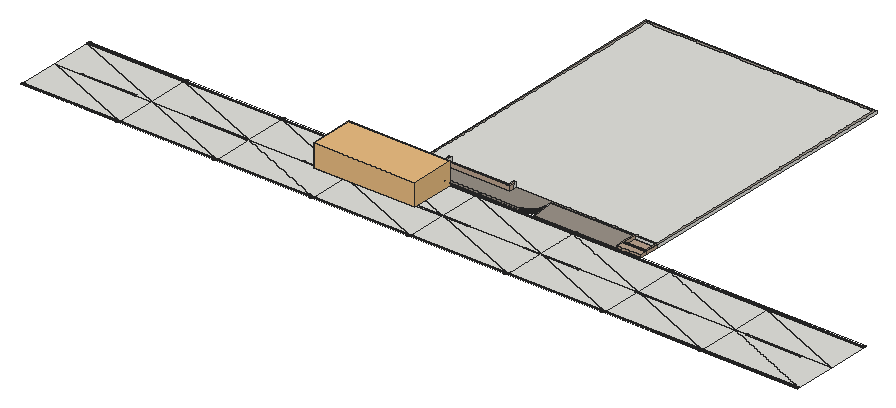
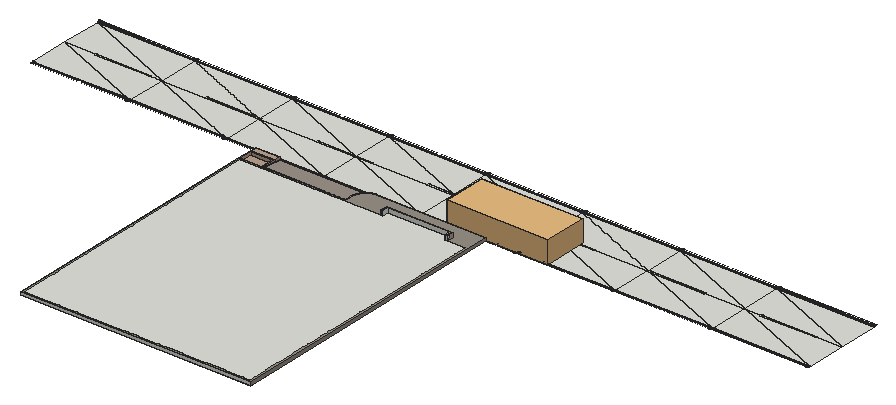
# SketchUp Ruby script. Lengths in inches.
U = 1.inch
M = Sketchup.active_model
def pt(a) = Geom::Point3d.new(a.map { |v| v * U })
def face(e, loops, mat)
  f = e.add_face(loops[0].map { |a| pt(a) })
  loops[1..].each { |l| e.add_face(l.map { |a| pt(a) }).erase! }
  f.material = f.back_material = mat if mat
  f
end
# faces: each face lists its corners as indices into pts; further lists are holes
def faces(e, pts, list, mat = nil) = list.each { |f| face(e, (f[0].is_a?(Array) ? f : [f]).map { |l| l.map { |i| pts[i] } }, mat) }
# xy, xz, yz: faces in a plane at the given z, y or x. An outline is a flat list of corners, or four numbers for a rectangle; further outlines are holes
def ring(l) = l.size == 4 ? [[l[0], l[1]], [l[2], l[1]], [l[2], l[3]], [l[0], l[3]]] : l.each_slice(2).to_a
def flat(e, list, mat, &to3) = list.each { |f| face(e, (f[0].is_a?(Array) ? f : [f]).map { |l| ring(l).map { |u, v| to3.(u, v) } }, mat) }
def xy(e, z, list, mat = nil) = flat(e, list, mat) { |x, y| [x, y, z] }
def xz(e, y, list, mat = nil) = flat(e, list, mat) { |x, z| [x, y, z] }
def yz(e, x, list, mat = nil) = flat(e, list, mat) { |y, z| [x, y, z] }
def lines(e, pts, list) = list.each { |a, b| e.add_line(pt(pts[a]), pt(pts[b])) }
# prism: a flat outline (further loops are holes) pulled along v
def prism(e, loops, v, mat = nil)
  f = face(e, loops, mat); d = Geom::Vector3d.new(v.map { |x| x * U })
  f.pushpull(f.normal.samedirection?(d) ? d.length : -d.length)
end
def box(e, o, s, mat = nil) = prism(e, [[o, [o[0] + s[0], o[1], o[2]], [o[0] + s[0], o[1] + s[1], o[2]], [o[0], o[1] + s[1], o[2]]]], [0, 0, s[2]], mat)
def at(x, y, z, deg = 0) = Geom::Transformation.translation(pt([x, y, z])) * Geom::Transformation.rotation(ORIGIN, Z_AXIS, deg.degrees)
def axes(o, x, y, z) = Geom::Transformation.new([*x, 0, *y, 0, *z, 0, *pt(o).to_a, 1])
def part(name) = M.definitions.add(name)
# library, detail: a bought-in or finely detailed component or shape, given as its bounding box
def library(name, o, s) = part(name).tap { |d| box(d.entities, o, s) }
def detail(e, o, s) = box(e.add_group.entities, o, s)
def put(e, d, t, mat = nil) = e.add_instance(d, t).tap { |i| i.material = mat if mat }
def group(e, t, mat = nil) = e.add_group.tap { |g| g.transformation = t; g.material = mat if mat }.entities
root = M.entities
M.materials.add("Sand Stones 01 100cm").color = [188, 164, 143]
M.materials.add("Tiles L02 200cm").color = [152, 144, 134]
c1 = library("Car 033",[-43.24,-98.19,-1.29],[86.48,201.64,57.79])
xy(root,0.19,[[0,119.84,0.61,119.84,0,120.23],[0.61,119.84,0.61,120.23,0,120.23],[0,281.6,0.66,281.6,0,281.84],[0.66,281.6,0.66,281.84,0,281.84],[0,281.84,0.66,281.84,0,285.35],
  [0.66,281.84,0.66,285.35,0,285.35],[0,285.35,0.66,285.35,0,285.61],[0.66,285.35,0.66,285.61,0,285.61]])
xz(root,115.97,[[0,-0.1,0,0.09,192.375,0.11],[0,-0.1,192.375,0.11,192.375,-0.07],[192.375,-0.07,192.375,0.11,384.75,-0.05],[384.75,-0.05,192.375,0.11,384.75,0.13],[384.75,-0.05,384.75,0.13,577.125,-0.03],
  [577.125,-0.03,384.75,0.13,577.125,0.15],[577.125,-0.03,577.125,0.15,769.5,-0.01],[769.5,-0.01,577.125,0.15,769.5,0.18],[769.5,-0.01,769.5,0.18,961.88,0.02],[961.88,0.02,769.5,0.18,961.88,0.2],
  [961.88,0.02,961.88,0.2,1154.25,0.04],[1154.25,0.04,961.88,0.2,1154.25,0.22],[1154.25,0.04,1154.25,0.22,1346.63,0.0625],[1346.63,0.0625,1154.25,0.22,1346.63,0.24],[1346.63,0.0625,1346.63,0.24,1539,0.27],
  [1346.63,0.0625,1539,0.27,1539,0.08]])
xz(root,116.08,[[0,-0.1,0.61,-0.1,0,0.09],[0.61,-0.1,0.61,0.09,0,0.09],[0.61,-0.1,192.375,-0.07,0.61,0.09],[192.375,-0.07,192.375,0.11,0.61,0.09],[192.375,-0.07,384.75,-0.05,384.75,0.13],
  [192.375,-0.07,384.75,0.13,192.375,0.11],[384.75,-0.05,577.125,-0.03,577.125,0.15],[384.75,-0.05,577.125,0.15,384.75,0.13],[577.125,-0.03,769.5,-0.01,769.5,0.18],[577.125,-0.03,769.5,0.18,577.125,0.15],
  [769.5,-0.01,961.875,0.02,961.875,0.2],[769.5,-0.01,961.875,0.2,769.5,0.18],[961.875,0.02,1154.25,0.04,1154.25,0.22],[961.875,0.02,1154.25,0.22,961.875,0.2],[1154.25,0.04,1346.625,0.0625,1346.625,0.24],
  [1154.25,0.04,1346.625,0.24,1154.25,0.22],[1346.625,0.0625,1538.36,0.08,1346.625,0.24],[1538.36,0.08,1538.36,0.27,1346.625,0.24],[1538.36,0.08,1539,0.08,1538.36,0.27],[1539,0.08,1539,0.27,1538.36,0.27]])
xz(root,120.55,[[0,-1.53,0,-0.19,0.61,-0.19],[0,-1.53,0.61,-0.19,0.61,-1.53],[0.61,-1.53,0.61,-0.19,192.375,-0.17],[0.61,-1.53,192.375,-0.17,192.375,-1.51],[192.375,-1.51,192.375,-0.17,384.75,-0.15],
  [192.375,-1.51,384.75,-0.15,384.75,-1.49],[384.75,-1.49,384.75,-0.15,577.125,-0.13],[384.75,-1.49,577.125,-0.13,577.125,-1.46],[577.125,-1.46,577.125,-0.13,769.5,-1.44],[769.5,-1.44,577.125,-0.13,769.5,-0.1],
  [769.5,-1.44,769.5,-0.1,961.875,-0.08],[769.5,-1.44,961.875,-0.08,961.875,-1.42],[961.875,-1.42,1154.25,-0.06,1154.25,-1.4],[961.875,-1.42,961.875,-0.08,1154.25,-0.06],[1154.25,-1.4,1154.25,-0.06,1346.625,-0.04],
  [1154.25,-1.4,1346.625,-0.04,1346.63,-1.375],[1346.63,-1.375,1346.625,-0.04,1538.36,-0.01],[1346.63,-1.375,1538.36,-0.01,1538.36,-1.35],[1538.36,-1.35,1538.36,-0.01,1539,-0.01],[1538.36,-1.35,1539,-0.01,1539,-1.35],
  [0,-0.19,0,-0.01,0.61,-0.01],[0,-0.19,0.61,-0.01,0.61,-0.19],[0.61,-0.19,0.61,-0.01,192.375,0.01],[0.61,-0.19,192.375,0.01,192.375,-0.17],[192.375,-0.17,192.375,0.01,384.75,-0.15],
  [384.75,-0.15,192.375,0.01,384.75,0.03],[384.75,-0.15,384.75,0.03,577.125,-0.13],[577.125,-0.13,384.75,0.03,577.125,0.06],[577.125,-0.13,577.125,0.06,769.5,0.08],[577.125,-0.13,769.5,0.08,769.5,-0.1],
  [769.5,-0.1,769.5,0.08,961.875,-0.08],[961.875,-0.08,769.5,0.08,961.875,0.1],[961.875,-0.08,961.875,0.1,1154.25,-0.06],[1154.25,-0.06,961.875,0.1,1154.25,0.125],[1154.25,-0.06,1154.25,0.125,1346.625,-0.04],
  [1346.625,-0.04,1154.25,0.125,1346.625,0.15],[1346.625,-0.04,1346.625,0.15,1538.36,0.17],[1346.625,-0.04,1538.36,0.17,1538.36,-0.01],[1538.36,-0.01,1538.36,0.17,1539,0.17],[1538.36,-0.01,1539,0.17,1539,-0.01]])
xz(root,281.28,[[0,-1.53,0.66,-1.53,0,-0.31],[0.66,-1.53,0.66,-0.31,0,-0.31],[0.66,-1.53,192.375,-1.51,0.66,-0.31],[192.375,-1.51,192.375,-0.28,0.66,-0.31],[192.375,-1.51,384.75,-0.26,192.375,-0.28],
  [192.375,-1.51,384.75,-1.49,384.75,-0.26],[384.75,-1.49,577.125,-0.24,384.75,-0.26],[384.75,-1.49,577.125,-1.47,577.125,-0.24],[577.125,-1.47,769.5,-1.44,577.125,-0.24],[769.5,-1.44,769.5,-0.22,577.125,-0.24],
  [769.5,-1.44,961.875,-0.19,769.5,-0.22],[769.5,-1.44,961.875,-1.42,961.875,-0.19],[961.875,-1.42,1154.25,-0.17,961.875,-0.19],[961.875,-1.42,1154.25,-1.4,1154.25,-0.17],[1154.25,-1.4,1346.63,-0.15,1154.25,-0.17],
  [1154.25,-1.4,1346.63,-1.38,1346.63,-0.15],[1346.63,-1.38,1538.23,-1.35,1346.63,-0.15],[1538.23,-1.35,1538.23,-0.125,1346.63,-0.15],[1538.23,-1.35,1539,-1.35,1538.23,-0.125],[1539,-1.35,1539,-0.125,1538.23,-0.125],
  [0,-0.31,0.66,-0.31,0,-0.01],[0.66,-0.31,0.66,-0.01,0,-0.01],[0.66,-0.31,192.375,-0.28,0.66,-0.01],[192.375,-0.28,192.375,0.01,0.66,-0.01],[192.375,-0.28,384.75,-0.26,192.375,0.01],
  [384.75,-0.26,384.75,0.03,192.375,0.01],[384.75,-0.26,577.125,-0.24,384.75,0.03],[577.125,-0.24,577.125,0.06,384.75,0.03],[577.125,-0.24,769.5,-0.22,769.5,0.08],[577.125,-0.24,769.5,0.08,577.125,0.06],
  [769.5,-0.22,961.875,-0.19,769.5,0.08],[961.875,-0.19,961.875,0.1,769.5,0.08],[961.875,-0.19,1154.25,-0.17,961.875,0.1],[1154.25,-0.17,1154.25,0.12,961.875,0.1],[1154.25,-0.17,1346.63,-0.15,1154.25,0.12],
  [1346.63,-0.15,1346.63,0.15,1154.25,0.12],[1346.63,-0.15,1538.23,-0.125,1346.63,0.15],[1538.23,-0.125,1538.23,0.17,1346.63,0.15],[1538.23,-0.125,1539,-0.125,1538.23,0.17],[1539,-0.125,1539,0.17,1538.23,0.17]])
xz(root,285.75,[[0,-0.12,0,0.08,0.66,0.08],[0,-0.12,0.66,0.08,0.66,-0.12],[0.66,-0.12,0.66,0.08,192.375,0.1],[0.66,-0.12,192.375,0.1,192.375,-0.1],[192.375,-0.1,192.375,0.1,384.75,-0.08],
  [384.75,-0.08,192.375,0.1,384.75,0.125],[384.75,-0.08,384.75,0.125,577.125,-0.05],[577.125,-0.05,384.75,0.125,577.125,0.15],[577.125,-0.05,577.125,0.15,769.5,-0.03],[769.5,-0.03,577.125,0.15,769.5,0.17],
  [769.5,-0.03,769.5,0.17,961.875,-0.01],[961.875,-0.01,769.5,0.17,961.875,0.19],[961.875,-0.01,961.875,0.19,1154.25,0.01],[1154.25,0.01,961.875,0.19,1154.25,0.22],[1154.25,0.01,1154.25,0.22,1346.63,0.04],
  [1346.63,0.04,1154.25,0.22,1346.625,0.24],[1346.63,0.04,1346.625,0.24,1538.23,0.26],[1346.63,0.04,1538.23,0.26,1538.23,0.06],[1538.23,0.06,1538.23,0.26,1539,0.26],[1538.23,0.06,1539,0.26,1539,0.06]])
p = [[0,200.91,-1.53],[0,120.55,-1.53],[192.375,120.55,-1.51],[192.375,200.91,-1.51],[384.75,120.55,-1.49],[384.75,200.91,-1.49],
  [577.125,120.55,-1.46],[577.125,200.91,-1.47],[769.5,120.55,-1.44],[769.5,200.91,-1.44],[161.27,199.56,-1.51],[161.27,202.27,-1.51],
  [51.47,202.27,-1.52],[51.47,199.56,-1.52],[380.88,199.56,-1.48],[380.88,202.27,-1.48],[271.08,202.27,-1.49],[271.08,199.56,-1.49],
  [600.49,199.56,-1.46],[600.49,202.27,-1.46],[490.6875,202.27,-1.47],[490.6875,199.56,-1.47],[0,281.28,-1.53],[192.375,281.28,-1.51],
  [384.75,281.28,-1.49],[577.125,281.28,-1.47],[769.5,281.28,-1.44],[961.875,120.55,-1.42],[961.875,200.91,-1.42],[1154.25,120.55,-1.4],
  [1154.25,200.91,-1.4],[1346.63,120.55,-1.375],[1346.63,200.91,-1.375],[1539,120.55,-1.35],[1539,200.91,-1.35],[820.1,199.56,-1.43],
  [820.1,202.27,-1.43],[710.3,202.27,-1.44],[710.3,199.56,-1.44],[1039.71,199.56,-1.4],[1039.71,202.27,-1.4],[929.91,202.27,-1.42],
  [929.91,199.56,-1.42],[1259.32,199.56,-1.38],[1259.32,202.27,-1.38],[1149.52,202.27,-1.39],[1149.52,199.56,-1.39],[1478.93,199.56,-1.35],
  [1478.93,202.27,-1.35],[1369.13,202.27,-1.37],[1369.13,199.56,-1.37],[961.875,281.28,-1.42],[1154.25,281.28,-1.4],[1346.63,281.28,-1.38],
  [1539,281.28,-1.35],[0,120.55,-0.01],[0,120.47,0.14],[0.61,120.47,0.14],[0.61,120.55,-0.01],[192.375,120.55,0.01],
  [192.375,120.47,0.17],[384.75,120.47,0.1875],[384.75,120.55,0.03],[577.125,120.47,0.21],[577.125,120.55,0.06],[0,281.36,0.14],
  [0,281.28,-0.01],[0.66,281.28,-0.01],[0.66,281.36,0.14],[192.375,281.28,0.01],[192.375,281.36,0.16],[384.75,281.28,0.03],
  [384.75,281.36,0.1875],[577.125,281.28,0.06],[192.375,115.83,0.22],[192.375,115.97,0.11],[0,115.97,0.09],[0,115.83,0.2],
  [384.75,115.83,0.24],[384.75,115.97,0.13],[577.125,115.83,0.26],[577.125,115.97,0.15],[0,116.21,0.2],[0,116.08,0.09],
  [0.61,116.08,0.09],[0.61,116.21,0.2],[192.375,116.08,0.11],[192.375,116.21,0.22],[384.75,116.08,0.13],[384.75,116.21,0.24],
  [577.125,116.08,0.15],[0,120.23,0.19],[0.61,120.23,0.19],[769.5,120.47,0.23],[769.5,120.55,0.08],[961.875,120.47,0.26],
  [961.875,120.55,0.1],[1154.25,120.47,0.28],[1154.25,120.55,0.125],[1346.625,120.47,0.3],[1346.625,120.55,0.15],[1538.36,120.47,0.32],
  [1538.36,120.55,0.17],[577.125,281.36,0.21],[769.5,281.28,0.08],[769.5,281.36,0.23],[961.875,281.28,0.1],[961.875,281.36,0.25],
  [1154.25,281.28,0.12],[1154.25,281.36,0.28],[1346.63,281.28,0.15],[1346.63,281.36,0.3],[1538.23,281.28,0.17],[1538.23,281.36,0.32],
  [0,281.6,0.19],[0.66,281.6,0.19],[0.66,285.61,0.19],[0.66,285.75,0.08],[0,285.75,0.08],[0,285.61,0.19],
  [192.375,285.61,0.21],[192.375,285.75,0.1],[384.75,285.61,0.24],[384.75,285.75,0.125],[577.125,285.61,0.26],[577.125,285.75,0.15],
  [769.5,285.61,0.28],[769.5,285.75,0.17],[769.5,115.83,0.29],[769.5,115.97,0.18],[961.88,115.83,0.31],[961.88,115.97,0.2],
  [577.125,116.21,0.26],[769.5,116.08,0.18],[769.5,116.21,0.29],[961.875,116.08,0.2],[0.61,116.39,0.2],[0.61,119.84,0.19],
  [0,119.84,0.19],[0,116.39,0.2],[192.375,116.39,0.22],[192.375,119.84,0.22],[192.375,120.23,0.22],[384.75,120.23,0.24],
  [577.125,120.23,0.26],[1539,120.47,0.32],[1539,120.55,0.17],[1539,281.28,0.17],[1539,281.36,0.32],[192.375,281.6,0.21],
  [384.75,281.6,0.24],[192.375,281.84,0.21],[0.66,281.84,0.19],[192.375,285.35,0.21],[0.66,285.35,0.19],[961.875,285.61,0.3],
  [961.875,285.75,0.19],[1154.25,285.61,0.33],[1154.25,285.75,0.22],[2295.1875,-533,0],[2295.1875,-536,0],[1790.2,-533,0],
  [1790.2,-536,0]]
faces(root,p,[[0,1,2],[2,3,0],[3,2,4],[4,5,3],[5,4,6],[6,7,5],[8,9,7],[7,6,8],
  [10,11,12],[12,13,10],[14,15,16],[16,17,14],[18,19,20],[20,21,18],[22,0,3],[3,23,22],
  [23,3,5],[5,24,23],[24,5,7],[7,25,24],[9,26,25],[25,7,9],[9,8,27],[27,28,9],
  [28,27,29],[29,30,28],[30,29,31],[31,32,30],[33,34,32],[32,31,33],[35,36,37],[37,38,35],
  [39,40,41],[41,42,39],[43,44,45],[45,46,43],[47,48,49],[49,50,47],[26,9,28],[28,51,26],
  [51,28,30],[30,52,51],[52,30,32],[32,53,52],[34,54,53],[53,32,34],[55,56,57],[57,58,55],
  [59,58,57],[57,60,59],[59,60,61],[61,62,59],[62,61,63],[63,64,62],[65,66,67],[67,68,65],
  [68,67,69],[69,70,68],[70,69,71],[71,72,70],[72,71,73],[74,75,76],[76,77,74],[78,79,75],
  [75,74,78],[80,81,79],[79,78,80],[82,83,84],[84,85,82],[85,84,86],[86,87,85],[87,86,88],
  [88,89,87],[89,88,90],[56,91,92],[92,57,56],[60,57,92],[64,63,93],[93,94,64],[94,93,95],
  [95,96,94],[96,95,97],[97,98,96],[98,97,99],[99,100,98],[100,99,101],[101,102,100],[73,103,72],
  [103,73,104],[104,105,103],[105,104,106],[106,107,105],[107,106,108],[108,109,107],[109,108,110],[110,111,109],
  [110,112,113],[113,111,110],[114,65,68],[68,115,114],[115,68,70],[116,117,118],[118,119,116],[120,121,117],
  [117,116,120],[122,123,121],[121,120,122],[124,125,123],[123,122,124],[126,127,125],[125,124,126],[128,129,81],
  [81,80,128],[130,131,129],[129,128,130],[90,132,89],[132,90,133],[133,134,132],[134,133,135],[136,137,138],
  [138,139,136],[140,141,137],[92,137,141],[141,142,92],[92,142,60],[60,142,143],[143,61,60],[61,143,144],
  [144,63,61],[102,101,145],[145,146,102],[113,112,147],[147,148,113],[70,149,115],[149,70,72],[72,150,149],
  [150,72,103],[149,151,152],[152,115,149],[151,153,154],[154,152,151],[116,154,153],[153,120,116],[155,156,127],
  [127,126,155],[157,158,156],[156,155,157]])
lines(root,p,[[159,160],[161,162]])
put(root,c1,axes([620.37,238.49,-0.47],[0,1,0],[-1,0,0],[0,0,0.76]))
g1 = group(root,at(672.95,472.76,0))
xy(g1,0,[[-36,-187.15,-36,396,420,396,420,-146,208.53,-146,208.53,-159.35,208.52,-159.64,208.51,-159.9375,208.5,-160.23,208.49,-160.52,208.47,-160.82,208.43,-161.4,208.4,-161.7,208.375,-161.99,208.34,-162.28,208.31,-162.57,208.27,-162.87,208.23,-163.16,208.03,-164.32,207.97,-164.61,207.91,-164.89,207.85,-165.18,207.78,-165.47,207.72,-165.75,207.64,-166.04,207.57,-166.32,207.49,-166.61,207.33,-167.17,207.24,-167.45,207.15,-167.74,207.06,-168.01,206.96,-168.29,206.87,-168.57,206.77,-168.85,206.66,-169.12,206.55,-169.4,206.22,-170.21,205.98,-170.75,205.85,-171.02,205.73,-171.28,205.6,-171.55,205.46,-171.81,205.33,-172.07,204.91,-172.85,204.61,-173.35,204.46,-173.61,204.31,-173.86,204.15,-174.11,203.99,-174.35,203.83,-174.6,203.67,-174.84,203.5,-175.09,203.16,-175.57,202.99,-175.8,202.8125,-176.04,202.63,-176.27,202.27,-176.73,202.08,-176.96,201.89,-177.1875,201.7,-177.41,201.51,-177.63,201.3125,-177.85,201.11,-178.07,200.91,-178.29,200.51,-178.71,200.3,-178.92,199.88,-179.33,199.66,-179.53,199.45,-179.73,199.01,-180.13,198.57,-180.51,198.11,-180.89,197.42,-181.43,197.18,-181.61,196.95,-181.78,196.71,-181.95,196.47,-182.125,196.22,-182.29,195.98,-182.45,195.73,-182.62,195.49,-182.77,195.24,-182.93,194.99,-183.08,194.73,-183.24,194.48,-183.38,194.22,-183.53,193.97,-183.67,193.71,-183.8125,193.45,-183.95,193.1875,-184.09,192.92,-184.22,192.66,-184.35,192.39,-184.47,192.13,-184.6,191.59,-184.84,191.32,-184.95,191.05,-185.07,190.77,-185.17,190.23,-185.39,189.67,-185.59,188.55,-185.95,187.99,-186.11,187.7,-186.19,187.42,-186.27,187.13,-186.34,186.85,-186.41,186.5625,-186.47,186.27,-186.53,185.99,-186.59,185.7,-186.65,184.54,-186.85,184.25,-186.89,183.95,-186.93,183.08,-187.02,182.78,-187.05,182.2,-187.09,181.9,-187.11,181.61,-187.125,181.32,-187.13,181.02,-187.14,180.73,-187.15]])
xy(g1,6,[[8.86,-153.04,131.14,-153.04,131.14,-141.14,415.14,-141.14,415.14,391.14,-31.14,391.14,-31.14,-141.14,8.86,-141.14]])
xy(g1,6,[[[-36,-187.15,180.73,-187.15,181.02,-187.14,181.32,-187.13,181.61,-187.125,181.9,-187.11,182.2,-187.09,182.78,-187.05,183.08,-187.02,183.95,-186.93,184.25,-186.89,184.54,-186.85,185.7,-186.65,185.99,-186.59,186.27,-186.53,186.5625,-186.47,186.85,-186.41,187.13,-186.34,187.42,-186.27,187.7,-186.19,187.99,-186.11,188.55,-185.95,189.67,-185.59,190.23,-185.39,190.77,-185.17,191.05,-185.07,191.32,-184.95,191.59,-184.84,192.13,-184.6,192.39,-184.47,192.66,-184.35,192.92,-184.22,193.1875,-184.09,193.45,-183.95,193.71,-183.8125,193.97,-183.67,194.22,-183.53,194.48,-183.38,194.73,-183.24,194.99,-183.08,195.24,-182.93,195.49,-182.77,195.73,-182.62,195.98,-182.45,196.22,-182.29,196.47,-182.125,196.71,-181.95,196.95,-181.78,197.18,-181.61,197.42,-181.43,198.11,-180.89,198.57,-180.51,199.01,-180.13,199.45,-179.73,199.66,-179.53,199.88,-179.33,200.3,-178.92,200.51,-178.71,200.91,-178.29,201.11,-178.07,201.3125,-177.85,201.51,-177.63,201.7,-177.41,201.89,-177.1875,202.08,-176.96,202.27,-176.73,202.63,-176.27,202.8125,-176.04,202.99,-175.8,203.16,-175.57,203.5,-175.09,203.67,-174.84,203.83,-174.6,203.99,-174.35,204.15,-174.11,204.31,-173.86,204.46,-173.61,204.61,-173.35,204.91,-172.85,205.33,-172.07,205.46,-171.81,205.6,-171.55,205.73,-171.28,205.85,-171.02,205.98,-170.75,206.22,-170.21,206.55,-169.4,206.66,-169.12,206.77,-168.85,206.87,-168.57,206.96,-168.29,207.06,-168.01,207.15,-167.74,207.24,-167.45,207.33,-167.17,207.49,-166.61,207.57,-166.32,207.64,-166.04,207.72,-165.75,207.78,-165.47,207.85,-165.18,207.91,-164.89,207.97,-164.61,208.03,-164.32,208.23,-163.16,208.27,-162.87,208.31,-162.57,208.34,-162.28,208.375,-161.99,208.4,-161.7,208.43,-161.4,208.47,-160.82,208.49,-160.52,208.5,-160.23,208.51,-159.9375,208.52,-159.64,208.53,-159.35,208.53,-146,420,-146,420,396,-36,396],[4,-155.71,4,-141.14,-31.14,-141.14,-31.14,391.14,415.14,391.14,415.14,-141.14,136,-141.14,136,-155.71]]],"Tiles L02 200cm")
xy(g1,14.9375,[[4,-155.71,136,-155.71,136,-141.14,131.14,-141.14,131.14,-153.04,8.86,-153.04,8.86,-141.14,4,-141.14]],"Sand Stones 01 100cm")
xz(g1,-187.15,[[-36,0,180.43,6],[180.43,0,180.73,6]],"Tiles L02 200cm")
xz(g1,-155.71,[[4,6,136,14.9375]],"Sand Stones 01 100cm")
xz(g1,-153.04,[[8.86,6,131.14,14.9375]])
xz(g1,-146,[[208.53,0,420,6]])
xz(g1,-141.14,[[4,6,8.86,14.9375],[131.14,6,136,14.9375]])
xz(g1,396,[[-36,0,420,6]])
yz(g1,-36,[[-187.15,0,396,6]],"Tiles L02 200cm")
yz(g1,4,[[-146,6,-141.14,14.9375]])
yz(g1,4,[[-155.71,6,-146,14.9375]],"Sand Stones 01 100cm")
yz(g1,8.86,[[-153.04,6,-141.14,14.9375]])
yz(g1,131.14,[[-153.04,6,-141.14,14.9375]])
yz(g1,136,[[-146,6,-141.14,14.9375]])
yz(g1,136,[[-155.71,6,-146,14.9375]],"Sand Stones 01 100cm")
yz(g1,208.53,[[-159.05,0,-146,6]])
yz(g1,208.53,[[-159.35,0,-159.05,6]],"Tiles L02 200cm")
yz(g1,420,[[-146,0,396,6]])
p = [[181.02,-187.14,6],[180.73,-187.15,6],[180.73,-187.15,0],[181.02,-187.14,0],[181.32,-187.13,6],[181.32,-187.13,0],
  [181.61,-187.125,6],[181.61,-187.125,0],[181.9,-187.11,6],[181.9,-187.11,0],[182.2,-187.09,6],[182.2,-187.09,0],
  [182.49,-187.07,6],[182.49,-187.07,0],[182.78,-187.05,6],[182.78,-187.05,0],[183.08,-187.02,6],[183.08,-187.02,0],
  [183.37,-186.99,6],[183.37,-186.99,0],[183.66,-186.96,6],[183.66,-186.96,0],[183.95,-186.93,6],[183.95,-186.93,0],
  [184.25,-186.89,6],[184.25,-186.89,0],[184.54,-186.85,6],[184.54,-186.85,0],[184.83,-186.8,6],[184.83,-186.8,0],
  [185.12,-186.75,6],[185.12,-186.75,0],[185.41,-186.7,6],[185.41,-186.7,0],[185.7,-186.65,6],[185.7,-186.65,0],
  [185.99,-186.59,6],[185.99,-186.59,0],[186.27,-186.53,6],[186.27,-186.53,0],[186.5625,-186.47,6],[186.5625,-186.47,0],
  [186.85,-186.41,6],[186.85,-186.41,0],[187.13,-186.34,6],[187.13,-186.34,0],[187.42,-186.27,6],[187.42,-186.27,0],
  [187.7,-186.19,6],[187.7,-186.19,0],[187.99,-186.11,6],[187.99,-186.11,0],[188.27,-186.03,6],[188.27,-186.03,0],
  [188.55,-185.95,6],[188.55,-185.95,0],[188.83,-185.86,6],[188.83,-185.86,0],[189.11,-185.77,6],[189.11,-185.77,0],
  [189.39,-185.68,6],[189.39,-185.68,0],[189.67,-185.59,6],[189.67,-185.59,0],[189.95,-185.49,6],[189.95,-185.49,0],
  [190.23,-185.39,6],[190.23,-185.39,0],[190.5,-185.28,6],[190.5,-185.28,0],[190.77,-185.17,6],[190.77,-185.17,0],
  [191.05,-185.07,6],[191.05,-185.07,0],[191.32,-184.95,6],[191.32,-184.95,0],[191.59,-184.84,6],[191.59,-184.84,0],
  [191.86,-184.72,6],[191.86,-184.72,0],[192.13,-184.6,6],[192.13,-184.6,0],[192.39,-184.47,6],[192.39,-184.47,0],
  [192.66,-184.35,6],[192.66,-184.35,0],[192.92,-184.22,6],[192.92,-184.22,0],[193.1875,-184.09,6],[193.1875,-184.09,0],
  [193.45,-183.95,6],[193.45,-183.95,0],[193.71,-183.8125,6],[193.71,-183.8125,0],[193.97,-183.67,6],[193.97,-183.67,0],
  [194.22,-183.53,6],[194.22,-183.53,0],[194.48,-183.38,6],[194.48,-183.38,0],[194.73,-183.24,6],[194.73,-183.24,0],
  [194.99,-183.08,6],[194.99,-183.08,0],[195.24,-182.93,6],[195.24,-182.93,0],[195.49,-182.77,6],[195.49,-182.77,0],
  [195.73,-182.62,6],[195.73,-182.62,0],[195.98,-182.45,6],[195.98,-182.45,0],[196.22,-182.29,6],[196.22,-182.29,0],
  [196.47,-182.125,6],[196.47,-182.125,0],[196.71,-181.95,6],[196.71,-181.95,0],[196.95,-181.78,6],[196.95,-181.78,0],
  [197.18,-181.61,6],[197.18,-181.61,0],[197.42,-181.43,6],[197.42,-181.43,0],[197.65,-181.25,6],[197.65,-181.25,0],
  [197.88,-181.07,6],[197.88,-181.07,0],[198.11,-180.89,6],[198.11,-180.89,0],[198.34,-180.7,6],[198.34,-180.7,0],
  [198.57,-180.51,6],[198.57,-180.51,0],[198.79,-180.32,6],[198.79,-180.32,0],[199.01,-180.13,6],[199.01,-180.13,0],
  [199.23,-179.93,6],[199.23,-179.93,0],[199.45,-179.73,6],[199.45,-179.73,0],[199.66,-179.53,6],[199.66,-179.53,0],
  [199.88,-179.33,6],[199.88,-179.33,0],[200.09,-179.125,6],[200.09,-179.125,0],[200.3,-178.92,6],[200.3,-178.92,0],
  [200.51,-178.71,6],[200.51,-178.71,0],[200.71,-178.5,6],[200.71,-178.5,0],[200.91,-178.29,6],[200.91,-178.29,0],
  [201.11,-178.07,6],[201.11,-178.07,0],[201.3125,-177.85,6],[201.3125,-177.85,0],[201.51,-177.63,6],[201.51,-177.63,0],
  [201.7,-177.41,6],[201.7,-177.41,0],[201.89,-177.1875,6],[201.89,-177.1875,0],[202.08,-176.96,6],[202.08,-176.96,0],
  [202.27,-176.73,6],[202.27,-176.73,0],[202.45,-176.5,6],[202.45,-176.5,0],[202.63,-176.27,6],[202.63,-176.27,0],
  [202.8125,-176.04,6],[202.8125,-176.04,0],[202.99,-175.8,6],[202.99,-175.8,0],[203.16,-175.57,6],[203.16,-175.57,0],
  [203.33,-175.33,6],[203.33,-175.33,0],[203.5,-175.09,6],[203.5,-175.09,0],[203.67,-174.84,6],[203.67,-174.84,0],
  [203.83,-174.6,6],[203.83,-174.6,0],[203.99,-174.35,6],[203.99,-174.35,0],[204.15,-174.11,6],[204.15,-174.11,0],
  [204.31,-173.86,6],[204.31,-173.86,0],[204.46,-173.61,6],[204.46,-173.61,0],[204.61,-173.35,6],[204.61,-173.35,0],
  [204.76,-173.1,6],[204.76,-173.1,0],[204.91,-172.85,6],[204.91,-172.85,0],[205.05,-172.59,6],[205.05,-172.59,0],
  [205.19,-172.33,6],[205.19,-172.33,0],[205.33,-172.07,6],[205.33,-172.07,0],[205.46,-171.81,6],[205.46,-171.81,0],
  [205.6,-171.55,6],[205.6,-171.55,0],[205.73,-171.28,6],[205.73,-171.28,0],[205.85,-171.02,6],[205.85,-171.02,0],
  [205.98,-170.75,6],[205.98,-170.75,0],[206.1,-170.48,6],[206.1,-170.48,0],[206.22,-170.21,6],[206.22,-170.21,0],
  [206.33,-169.94,6],[206.33,-169.94,0],[206.44,-169.67,6],[206.44,-169.67,0],[206.55,-169.4,6],[206.55,-169.4,0],
  [206.66,-169.12,6],[206.66,-169.12,0],[206.77,-168.85,6],[206.77,-168.85,0],[206.87,-168.57,6],[206.87,-168.57,0],
  [206.96,-168.29,6],[206.96,-168.29,0],[207.06,-168.01,6],[207.06,-168.01,0],[207.15,-167.74,6],[207.15,-167.74,0],
  [207.24,-167.45,6],[207.24,-167.45,0],[207.33,-167.17,6],[207.33,-167.17,0],[207.41,-166.89,6],[207.41,-166.89,0],
  [207.49,-166.61,6],[207.49,-166.61,0],[207.57,-166.32,6],[207.57,-166.32,0],[207.64,-166.04,6],[207.64,-166.04,0],
  [207.72,-165.75,6],[207.72,-165.75,0],[207.78,-165.47,6],[207.78,-165.47,0],[207.85,-165.18,6],[207.85,-165.18,0],
  [207.91,-164.89,6],[207.91,-164.89,0],[207.97,-164.61,6],[207.97,-164.61,0],[208.03,-164.32,6],[208.03,-164.32,0],
  [208.08,-164.03,6],[208.08,-164.03,0],[208.13,-163.74,6],[208.13,-163.74,0],[208.18,-163.45,6],[208.18,-163.45,0],
  [208.23,-163.16,6],[208.23,-163.16,0],[208.27,-162.87,6],[208.27,-162.87,0],[208.31,-162.57,6],[208.31,-162.57,0],
  [208.34,-162.28,6],[208.34,-162.28,0],[208.375,-161.99,6],[208.375,-161.99,0],[208.4,-161.7,6],[208.4,-161.7,0],
  [208.43,-161.4,6],[208.43,-161.4,0],[208.45,-161.11,6],[208.45,-161.11,0],[208.47,-160.82,6],[208.47,-160.82,0],
  [208.49,-160.52,6],[208.49,-160.52,0],[208.5,-160.23,6],[208.5,-160.23,0],[208.51,-159.9375,6],[208.51,-159.9375,0],
  [208.52,-159.64,6],[208.52,-159.64,0],[208.53,-159.35,6],[208.53,-159.35,0]]
faces(g1,p,[[0,1,2,3],[4,0,3,5],[6,4,5,7],[8,6,7,9],[10,8,9,11],[12,10,11,13],[14,12,13,15],[16,14,15,17],
  [18,16,17,19],[20,18,19,21],[22,20,21,23],[24,22,23,25],[26,24,25,27],[28,26,27,29],[30,28,29,31],[32,30,31,33],
  [34,32,33,35],[36,34,35,37],[38,36,37,39],[40,38,39,41],[42,40,41,43],[44,42,43,45],[46,44,45,47],[48,46,47,49],
  [50,48,49,51],[52,50,51,53],[54,52,53,55],[56,54,55,57],[58,56,57,59],[60,58,59,61],[62,60,61,63],[64,62,63,65],
  [66,64,65,67],[68,66,67,69],[70,68,69,71],[72,70,71,73],[74,72,73,75],[76,74,75,77],[78,76,77,79],[80,78,79,81],
  [82,80,81,83],[84,82,83,85],[86,84,85,87],[88,86,87,89],[90,88,89,91],[92,90,91,93],[94,92,93,95],[96,94,95,97],
  [98,96,97,99],[100,98,99,101],[102,100,101,103],[104,102,103,105],[106,104,105,107],[108,106,107,109],[110,108,109,111],[112,110,111,113],
  [114,112,113,115],[116,114,115,117],[118,116,117,119],[120,118,119,121],[122,120,121,123],[124,122,123,125],[126,124,125,127],[128,126,127,129],
  [130,128,129,131],[132,130,131,133],[134,132,133,135],[136,134,135,137],[138,136,137,139],[140,138,139,141],[142,140,141,143],[144,142,143,145],
  [146,144,145,147],[148,146,147,149],[150,148,149,151],[152,150,151,153],[154,152,153,155],[156,154,155,157],[158,156,157,159],[160,158,159,161],
  [162,160,161,163],[164,162,163,165],[166,164,165,167],[168,166,167,169],[170,168,169,171],[172,170,171,173],[174,172,173,175],[176,174,175,177],
  [178,176,177,179],[180,178,179,181],[182,180,181,183],[184,182,183,185],[186,184,185,187],[188,186,187,189],[190,188,189,191],[192,190,191,193],
  [194,192,193,195],[196,194,195,197],[198,196,197,199],[200,198,199,201],[202,200,201,203],[204,202,203,205],[206,204,205,207],[208,206,207,209],
  [210,208,209,211],[212,210,211,213],[214,212,213,215],[216,214,215,217],[218,216,217,219],[220,218,219,221],[222,220,221,223],[224,222,223,225],
  [226,224,225,227],[228,226,227,229],[230,228,229,231],[232,230,231,233],[234,232,233,235],[236,234,235,237],[238,236,237,239],[240,238,239,241],
  [242,240,241,243],[244,242,243,245],[246,244,245,247],[248,246,247,249],[250,248,249,251],[252,250,251,253],[254,252,253,255],[256,254,255,257],
  [258,256,257,259],[260,258,259,261],[262,260,261,263],[264,262,263,265],[266,264,265,267],[268,266,267,269],[270,268,269,271],[272,270,271,273],
  [274,272,273,275],[276,274,275,277],[278,276,277,279],[280,278,279,281],[282,280,281,283],[284,282,283,285],[286,284,285,287],[288,286,287,289],
  [290,288,289,291],[292,290,291,293],[294,292,293,295],[296,294,295,297]],"Tiles L02 200cm")
g2 = group(root,at(881.47,285.61,0),"Tiles L02 200cm")
prism(g2,[[[163.65,29,0],[163.65,41.15,0],[163.65,41.15,6],[163.65,0,0.72]]],[-163.65,0,0],"Tiles L02 200cm")
g3 = group(root,at(1047.75,299.01,0),"Sand Stones 01 100cm")
xy(g3,0,[[-2.25,-13.26,45.2,0],[-2.25,0,45.2,27.75]])
xy(g3,0.4375,[[0.45,2.7,42.49,27.75]])
xy(g3,5.9375,[[-2.25,-13.26,45.2,0],[-2.25,0,45.2,0,45.2,27.75,42.49,27.75,42.49,2.7,0.45,2.7,0.45,27.75,-2.25,27.75]])
xz(g3,-13.26,[[-2.25,0,45.2,5.9375]])
xz(g3,0,[[-2.25,0,45.2,5.9375]])
xz(g3,2.7,[[0.45,0.4375,42.49,5.9375]])
xz(g3,27.75,[[-2.25,0,-2.25,5.9375,0.45,5.9375,0.45,0.4375,42.49,0.4375,42.49,5.9375,45.2,5.9375,45.2,0]])
yz(g3,-2.25,[[-13.26,0,0,5.9375],[0,0,27.75,5.9375]])
yz(g3,0.45,[[2.7,0.4375,27.75,5.9375]])
yz(g3,42.49,[[2.7,0.4375,27.75,5.9375]])
yz(g3,45.2,[[-13.26,0,0,5.9375],[0,0,27.75,5.9375]])
